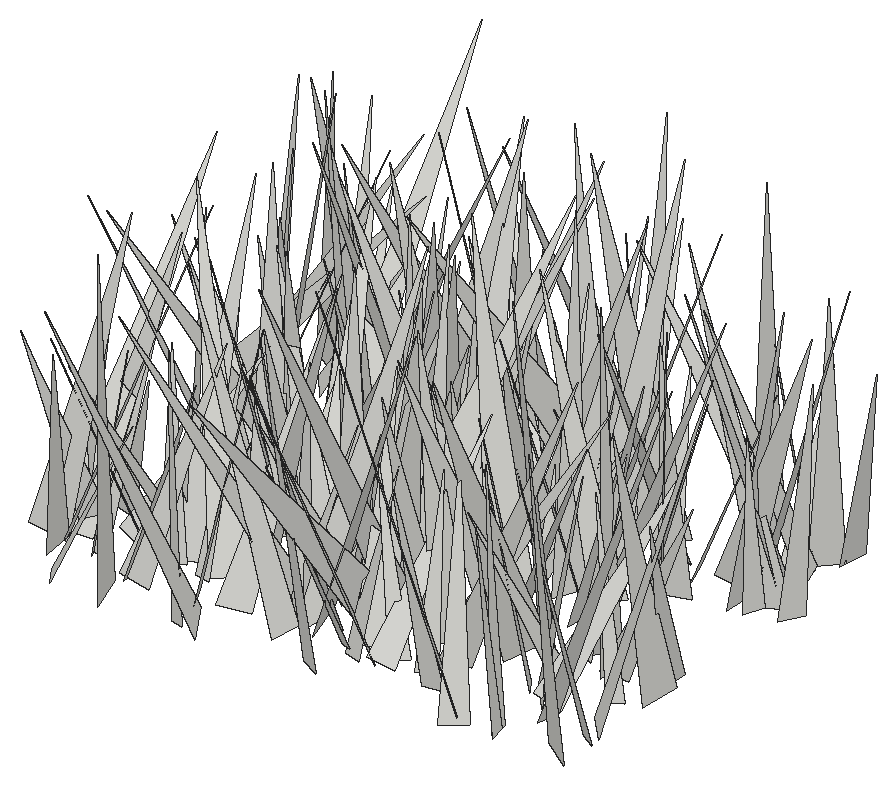
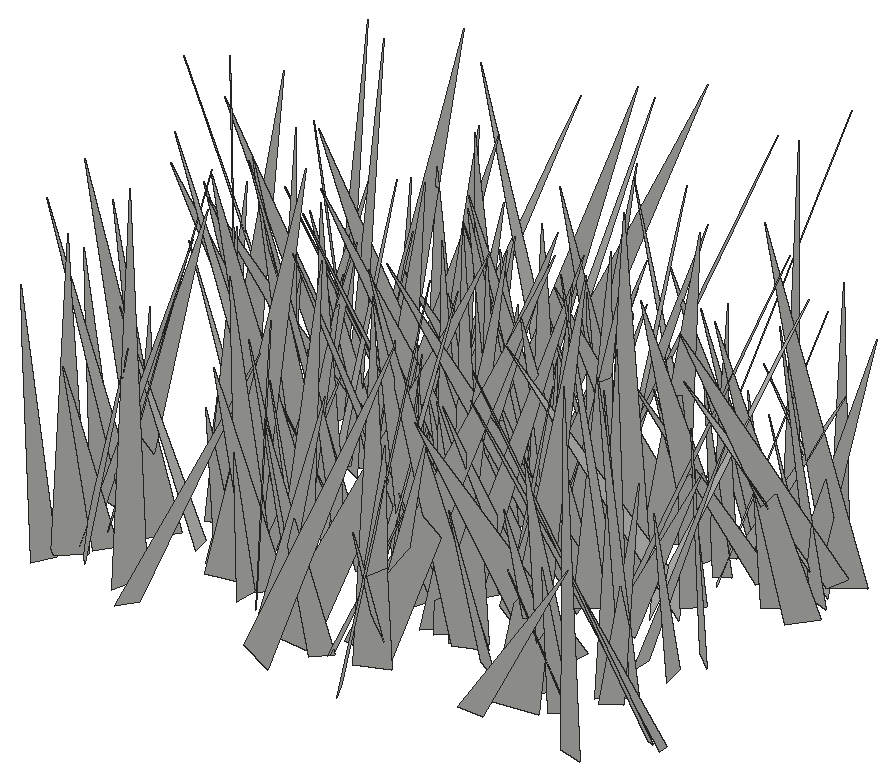
# SketchUp Ruby script. Lengths in inches.
U = 1.inch
M = Sketchup.active_model
def pt(a) = Geom::Point3d.new(a.map { |v| v * U })
def face(e, loops, mat)
  f = e.add_face(loops[0].map { |a| pt(a) })
  loops[1..].each { |l| e.add_face(l.map { |a| pt(a) }).erase! }
  f.material = f.back_material = mat if mat
  f
end
# faces: each face lists its corners as indices into pts; further lists are holes
def faces(e, pts, list, mat = nil) = list.each { |f| face(e, (f[0].is_a?(Array) ? f : [f]).map { |l| l.map { |i| pts[i] } }, mat) }
# xy, xz, yz: faces in a plane at the given z, y or x. An outline is a flat list of corners, or four numbers for a rectangle; further outlines are holes
def ring(l) = l.size == 4 ? [[l[0], l[1]], [l[2], l[1]], [l[2], l[3]], [l[0], l[3]]] : l.each_slice(2).to_a
def flat(e, list, mat, &to3) = list.each { |f| face(e, (f[0].is_a?(Array) ? f : [f]).map { |l| ring(l).map { |u, v| to3.(u, v) } }, mat) }
def xy(e, z, list, mat = nil) = flat(e, list, mat) { |x, y| [x, y, z] }
def xz(e, y, list, mat = nil) = flat(e, list, mat) { |x, z| [x, y, z] }
def yz(e, x, list, mat = nil) = flat(e, list, mat) { |y, z| [x, y, z] }
def lines(e, pts, list) = list.each { |a, b| e.add_line(pt(pts[a]), pt(pts[b])) }
# prism: a flat outline (further loops are holes) pulled along v
def prism(e, loops, v, mat = nil)
  f = face(e, loops, mat); d = Geom::Vector3d.new(v.map { |x| x * U })
  f.pushpull(f.normal.samedirection?(d) ? d.length : -d.length)
end
def box(e, o, s, mat = nil) = prism(e, [[o, [o[0] + s[0], o[1], o[2]], [o[0] + s[0], o[1] + s[1], o[2]], [o[0], o[1] + s[1], o[2]]]], [0, 0, s[2]], mat)
def at(x, y, z, deg = 0) = Geom::Transformation.translation(pt([x, y, z])) * Geom::Transformation.rotation(ORIGIN, Z_AXIS, deg.degrees)
def axes(o, x, y, z) = Geom::Transformation.new([*x, 0, *y, 0, *z, 0, *pt(o).to_a, 1])
def part(name) = M.definitions.add(name)
# library, detail: a bought-in or finely detailed component or shape, given as its bounding box
def library(name, o, s) = part(name).tap { |d| box(d.entities, o, s) }
def detail(e, o, s) = box(e.add_group.entities, o, s)
def put(e, d, t, mat = nil) = e.add_instance(d, t).tap { |i| i.material = mat if mat }
def group(e, t, mat = nil) = e.add_group.tap { |g| g.transformation = t; g.material = mat if mat }.entities
root = M.entities
c1 = part("fur_instance\#9")
p = [[0.8125,0,1.79],[0.67,-0.02,1.48],[0,-0.11,0],[0,0.11,0]]
faces(c1.entities,p,[[0,1,2,3]])
put(root,c1,axes([534.78,5.64,-21.86],[-6.5639,-4.29471,0.69968],[-4.06333,6.50273,1.7952],[1.55674,-1.13527,7.63588]))
put(root,c1,axes([530.92,5.27,-21.86],[6.72646,1.81373,2.96578],[2.30607,-7.16166,-0.85049],[-2.60144,-1.65881,6.91459]))
put(root,c1,axes([540.06,9.92,-21.86],[5.96387,-5.74764,0.45925],[-4.68382,-5.21453,-4.43673],[-3.36276,-2.93042,6.99418]))
put(root,c1,axes([540.83,7.86,-21.86],[-4.50054,-5.78959,0.45114],[-5.68851,4.51005,1.13049],[1.1678,-0.3432,7.24542]))
put(root,c1,axes([550.6875,6.2,-21.86],[-3.10043,-5.65859,2.0595],[-5.81568,3.41455,0.62657],[1.56175,1.48157,6.42182]))
put(root,c1,axes([527.36,6.95,-21.86],[5.21183,-0.69159,1.00189],[-0.40075,-5.13378,-1.45906],[-1.14955,-1.3458,5.051]))
put(root,c1,axes([528.53,5.1,-21.86],[3.11612,2.14822,0.04863],[2.13222,-3.08072,-0.53874],[0.26618,-0.47091,3.74631]))
put(root,c1,axes([539.89,5.63,-21.86],[-3.61019,-4.99925,2.09321],[-5.40705,3.49453,-0.97958],[0.37125,2.28107,6.08822]))
put(root,c1,axes([536.85,9.12,-21.86],[-6.99156,-3.62516,0.34789],[-3.32905,6.6672,2.57109],[1.47657,-2.13338,7.444]))
put(root,c1,axes([548.125,6.03,-21.86],[-3.70453,-1.18645,1.17686],[-1.32576,3.8289,-0.31316],[1.01735,0.66938,3.87726]))
put(root,c1,axes([546.48,5.59,-21.86],[-3.13208,3.88614,1.48189],[4.03166,3.29255,-0.11327],[1.02167,-1.07935,4.98991]))
put(root,c1,axes([534.21,5.15,-21.86],[2.11114,4.26728,1.69749],[4.08085,-2.60007,1.46097],[-2.10662,-0.76029,4.53125]))
put(root,c1,axes([544.27,7.17,-21.86],[0.17037,-4.40384,1.04145],[-4.5148,-0.2364,-0.26107],[-0.30825,1.02847,4.3994]))
put(root,c1,axes([545.93,6.41,-21.86],[-6.31099,-5.2237,1.0112],[-5.28027,5.95593,-2.18722],[-0.65451,2.31907,7.89505]))
put(root,c1,axes([533.68,6.97,-21.86],[5.91305,2.63208,1.30513],[2.84881,-5.85376,-1.10147],[-0.71801,-1.54954,6.37799]))
put(root,c1,axes([547.97,6.27,-21.86],[-4.75488,-0.89522,1.48594],[-1.16705,4.85843,-0.80746],[1.28353,1.10117,4.77057]))
put(root,c1,axes([539.92,7.66,-21.86],[-2.11494,-3.26023,0.3236],[-3.25153,2.04149,-0.68318],[-0.40176,0.64034,3.82562]))
put(root,c1,axes([530.75,6.95,-21.86],[4.6292,0.17151,0.50537],[0.17521,-4.6565,-0.02456],[-0.5041,-0.0434,4.63231]))
put(root,c1,axes([531.11,6.63,-21.86],[-0.2633,5.21725,2.01289],[5.21535,0.95622,-1.79623],[2.01778,-1.79073,4.90536]))
put(root,c1,axes([527.55,8.98,-21.86],[3.42862,-3.42654,1.21049],[-3.04602,-3.61734,-1.61199],[-1.98197,-0.36822,4.57144]))
put(root,c1,axes([550.95,7.64,-21.86],[-3.27995,-3.84872,1.10692],[-4.00472,3.15616,-0.89264],[0.01123,1.42196,4.97734]))
put(root,c1,axes([538.19,8.56,-21.86],[7.97506,1.59703,0.67128],[1.71117,-7.75527,-1.87893],[-0.27022,-1.97686,7.91339]))
put(root,c1,axes([537.64,7.04,-21.86],[-7.05219,-0.0174,0.36445],[-0.04272,7.04446,-0.49029],[0.36236,0.49184,7.03515]))
put(root,c1,axes([530.27,10.26,-21.86],[-4.13321,-3.41194,0.20507],[-3.07913,3.85633,2.10107],[1.48403,-1.5014,4.93054]))
put(root,c1,axes([540.35,10.58,-21.86],[0.33917,-8.30019,0.61155],[-8.21231,-0.43312,-1.32383],[-1.35096,0.54903,8.20095]))
put(root,c1,axes([530.93,7.98,-21.86],[-3.23089,-3.2407,0.20186],[-3.09319,2.98531,-1.58167],[-0.98745,1.25194,4.29408]))
put(root,c1,axes([526.48,7.53,-21.86],[1.86303,-6.4471,2.90273],[-6.99316,-1.23765,1.73947],[1.04242,3.21946,6.48153]))
put(root,c1,axes([538.75,8.64,-21.86],[-2.94659,-4.28728,0.79485],[-4.35538,2.84813,-0.78348],[-0.2081,1.09651,5.14289]))
put(root,c1,axes([545.16,11.39,-21.86],[6.488,-4.94571,0.82766],[-4.48999,-6.33233,-2.64212],[-2.23271,-1.63731,7.71838]))
put(root,c1,axes([542.06,8.05,-21.86],[-1.79664,3.17113,0.9039],[3.29721,1.71578,0.53432],[-0.03822,-1.04932,3.60534]))
put(root,c1,axes([528.65,7.34,-21.86],[2.93854,2.24557,1.05284],[2.03507,-3.11619,0.96641],[-1.41759,0.18132,3.56983]))
put(root,c1,axes([547.59,9.15,-21.86],[4.29125,3.34973,1.68987],[3.74545,-3.97458,-1.63261],[-0.21889,-2.33948,5.19327]))
put(root,c1,axes([538.01,8.5,-21.86],[-4.77809,0.40303,0.49366],[0.4272,4.79644,0.21897],[0.47289,-0.2608,4.79006]))
put(root,c1,axes([537.06,8.1,-21.86],[2.48119,3.58815,0.88423],[3.68479,-2.32113,-0.92071],[0.2811,-1.24521,4.2642]))
put(root,c1,axes([543.37,7.96,-21.86],[-2.54986,2.80817,1.27437],[2.87177,2.76487,-0.34653],[1.12374,-0.69377,3.77724]))
put(root,c1,axes([538.08,10.45,-21.86],[2.95419,-3.46444,1.08183],[-2.95275,-3.10527,-1.88109],[-2.11044,-0.50488,4.14621]))
put(root,c1,axes([531.36,8.52,-21.86],[1.67153,-3.68103,1.97281],[-4.08391,-1.88531,-0.05752],[-0.87388,1.76964,4.04237]))
put(root,c1,axes([528.93,7.34,-21.86],[1.45638,3.8911,0.37542],[3.87774,-1.48869,0.38679],[-0.49475,-0.21394,4.13668]))
put(root,c1,axes([546.92,10.95,-21.86],[-4.05266,-1.43323,0.72397],[-1.06557,3.87082,1.69814],[1.20119,-1.40176,3.94899]))
put(root,c1,axes([546.9,9.44,-21.86],[-3.48684,-2.54111,1.02639],[-2.66037,3.53733,-0.28017],[0.65812,0.83597,4.30544]))
put(root,c1,axes([526.6,9.09,-21.86],[2.41252,4.65389,1.89869],[5.02303,-2.30836,-0.72433],[-0.1815,-2.02404,5.19175]))
put(root,c1,axes([530.49,9.68,-21.86],[0.50859,-3.54434,0.97529],[-3.61365,-0.30136,0.78924],[0.67458,1.05784,3.49258]))
put(root,c1,axes([540.58,8.12,-21.86],[-2.22109,4.73282,1.14399],[4.81333,2.32397,-0.26934],[0.73496,-0.91711,5.22114]))
put(root,c1,axes([542.74,10.16,-21.86],[3.54462,-5.56954,2.15269],[-5.7416,-3.86654,-0.54956],[-1.63946,1.49942,6.57891]))
put(root,c1,axes([527.76,10.34,-21.86],[0.50493,-3.90237,0.56248],[-3.75126,-0.30094,1.27958],[1.21364,0.69337,3.72104]))
put(root,c1,axes([541.68,7.43,-21.86],[-1.38897,4.86037,0.26759],[4.61521,1.40338,-1.53442],[1.54748,0.17706,4.81643]))
put(root,c1,axes([534.17,9.83,-21.86],[6.74375,-1.56753,0.95704],[-1.61805,-6.79399,0.27364],[-0.86892,0.48558,6.91813]))
put(root,c1,axes([532.88,8.29,-21.86],[1.32341,3.79294,0.4756],[3.74321,-1.38791,0.65276],[-0.77522,-0.22654,3.9638]))
put(root,c1,axes([534.07,11.92,-21.86],[-4.79038,-5.44103,1.36632],[-5.2062,4.98101,1.5825],[2.08977,-0.06337,7.07448]))
put(root,c1,axes([543.89,8.81,-21.86],[6.12264,-2.56902,1.18593],[-2.80714,-5.86992,1.77677],[-0.35534,2.10644,6.39763]))
put(root,c1,axes([543.74,12.12,-21.86],[4.33462,-5.23656,1.50263],[-4.77333,-4.57611,-2.17783],[-2.62578,-0.3257,6.43953]))
put(root,c1,axes([548.82,8.06,-21.86],[6.71372,1.26121,1.18447],[0.98901,-6.69183,1.51954],[-1.41968,1.3025,6.66001]))
put(root,c1,axes([540.61,7.15,-21.86],[3.46655,5.88623,0.70358],[5.62008,-3.5225,1.77941],[-1.8861,0.32244,6.59533]))
put(root,c1,axes([536.04,9.95,-21.86],[0.99186,4.25892,2.03749],[4.71935,-0.95274,-0.30591],[-0.13232,-2.05608,4.36218]))
put(root,c1,axes([533.63,9.02,-21.86],[-4.74257,5.72398,1.5327],[5.90767,4.72004,0.65254],[0.46105,-1.60076,7.40474]))
put(root,c1,axes([550.99,11.6875,-21.86],[5.89812,-2.41371,1.85981],[-1.99813,-6.12286,-1.60962],[-2.30052,-0.87028,6.16628]))
put(root,c1,axes([550.64,8.54,-21.86],[5.3088,5.05785,1.00754],[5.10033,-5.36326,0.04959],[-0.76398,-0.65873,7.33231]))
put(root,c1,axes([535.15,7.22,-21.86],[-4.70627,4.28235,1.06672],[3.70191,4.67966,-2.45399],[2.40255,1.178,5.87073]))
put(root,c1,axes([540.34,11.71,-21.86],[-4.48343,0.78051,2.64752],[1.64873,4.80743,1.37477],[2.21365,-1.99978,4.33824]))
put(root,c1,axes([545.76,11.88,-21.86],[-3.953,-6.85404,2.35159],[-6.87911,4.39144,1.23577],[2.27722,1.36799,7.81517]))
put(root,c1,axes([529.01,9.04,-21.86],[0.32449,4.79651,0.65441],[4.29347,0.01783,-2.25961],[2.23626,-0.73022,4.24334]))
put(root,c1,axes([548.07,8.9375,-21.86],[-0.77489,5.32124,0.74593],[4.8544,1.01638,-2.20776],[2.30365,-0.35187,4.90325]))
put(root,c1,axes([529.91,12.04,-21.86],[2.72527,-3.47225,0.02549],[-3.46346,-2.7159,0.33551],[0.24824,0.22715,4.40125]))
put(root,c1,axes([536.96,11.52,-21.86],[3.71508,-1.29272,0.27873],[-1.28155,-3.72443,-0.19222],[-0.32626,-0.0905,3.92887]))
put(root,c1,axes([526.21,10.46,-21.86],[3.16186,-4.77933,2.12939],[-5.21892,-2.70344,1.68164],[0.37303,2.68757,5.47827]))
put(root,c1,axes([527.26,7.59,-21.86],[5.40862,3.75774,0.29196],[3.28966,-4.95573,2.84217],[-1.83956,2.18614,5.94103]))
put(root,c1,axes([550.65,12.85,-21.86],[4.29129,-1.7599,0.57931],[-1.53313,-4.1935,-1.38278],[-1.04037,-1.07949,4.42723]))
put(root,c1,axes([550,10.38,-21.86],[-0.43735,3.78387,0.74816],[3.7266,0.2203,1.06426],[-0.99494,-0.83814,3.65736]))
put(root,c1,axes([538.03,12.92,-21.86],[2.29516,-7.21123,1.1617],[-7.23425,-2.07612,1.40519],[1.00849,1.5189,7.43607]))
put(root,c1,axes([531.05,13.0625,-21.86],[-5.75391,-4.14909,0.07824],[-4.14913,5.75437,0.02082],[0.07564,0.02888,7.0938]))
put(root,c1,axes([548.73,11.93,-21.86],[2.75762,-4.13306,0.47465],[-3.98702,-2.46295,1.71739],[1.18791,1.32801,4.66232]))
put(root,c1,axes([531.58,8.9375,-21.86],[-5.90287,3.96424,1.22936],[3.5461,5.92766,-2.08769],[2.15678,1.10365,6.7971]))
put(root,c1,axes([542.28,11.16,-21.86],[4.10846,4.74791,0.21399],[4.46685,-3.7608,-2.31765],[1.62348,-1.66782,5.83529]))
put(root,c1,axes([543.86,12.18,-21.86],[5.27208,0.02621,0.0042],[0.02652,-5.23568,-0.61848],[-0.0011,-0.61849,5.23574]))
put(root,c1,axes([527.07,8.03,-21.86],[-5.0261,5.87636,0.71878],[5.2638,4.86732,-2.98524],[2.70938,1.44485,7.13314]))
put(root,c1,axes([533.44,13.21,-21.86],[2.7716,-4.32676,0.73791],[-4.29866,-2.85215,-0.57784],[-0.88707,0.30254,5.10575]))
put(root,c1,axes([536.59,12.125,-21.86],[-1.98157,5.41612,3.08152],[6.10168,2.34277,-0.19399],[1.26474,-2.81671,5.76397]))
put(root,c1,axes([536.55,10.88,-21.86],[0.16131,6.95669,2.04491],[7.08472,0.28432,-1.5261],[1.54396,-2.03146,6.78915]))
put(root,c1,axes([538.43,11.3,-21.86],[-1.99924,6.11191,2.2816],[6.3463,2.375,-0.80119],[1.51181,-1.88733,6.38047]))
put(root,c1,axes([532.84,12.125,-21.86],[5.17413,-4.7343,3.23528],[-5.24163,-5.67192,0.08293],[-2.32507,2.25121,7.01272]))
put(root,c1,axes([535.25,12.21,-21.86],[-4.86777,3.35697,1.6535],[3.6105,4.92638,0.62739],[0.98366,-1.46972,5.8797]))
put(root,c1,axes([530.53,16.49,-21.86],[-6.95908,-3.88864,0.42907],[-3.38575,6.42493,3.31533],[1.96017,-2.70799,7.24975]))
put(root,c1,axes([548.41,12.17,-21.86],[-6.67663,-0.80436,2.4344],[-1.05353,7.05179,-0.55944],[2.33738,0.88086,6.7016]))
put(root,c1,axes([549.54,13.53,-21.86],[6.08028,3.66314,2.96745],[4.34842,-6.22849,-1.22118],[-1.82087,-2.64225,6.99265]))
put(root,c1,axes([532.6875,14.28,-21.86],[4.51111,-4.76568,1.07484],[-4.75985,-4.61702,-0.49408],[-1.1004,0.43419,6.54353]))
put(root,c1,axes([546.88,12.46,-21.86],[2.00613,4.44684,1.43472],[4.67253,-1.91449,-0.59961],[-0.01581,-1.5549,4.84142]))
put(root,c1,axes([535.28,13.72,-21.86],[3.93197,-0.07434,1.3447],[0.21137,-4.06439,-0.84276],[-1.33006,-0.86567,3.84131]))
put(root,c1,axes([543.21,13.45,-21.86],[-2.98198,-2.20876,0.85448],[-2.34628,2.94214,-0.58291],[0.32208,0.98295,3.66484]))
put(root,c1,axes([545.26,14.48,-21.86],[6.29896,-1.22347,0.37639],[-1.1888,-6.29213,-0.55798],[-0.47466,-0.47719,6.39237]))
put(root,c1,axes([539.03,12.3,-21.86],[-6.72767,0.28008,1.7782],[-0.11729,6.79671,-1.51427],[1.7963,1.49276,6.56102]))
put(root,c1,axes([535.36,12.83,-21.86],[3.71678,-0.58843,1.31141],[-0.99782,-3.67326,1.17982],[-1.0346,1.42876,3.57333]))
put(root,c1,axes([543.28,16.53,-21.86],[-4.09949,-5.26965,1.04192],[-4.89422,4.20438,2.00758],[2.21389,-0.46331,6.36747]))
put(root,c1,axes([540.02,12.07,-21.86],[-6.09704,1.94582,1.05535],[1.61207,6.02238,-1.79053],[1.51697,1.42075,6.14444]))
put(root,c1,axes([539.18,14.87,-21.86],[-3.57828,-1.18752,0.86435],[-1.11493,3.67791,0.43741],[0.95617,-0.15551,3.74473]))
put(root,c1,axes([542.14,14.3125,-21.86],[-5.03128,5.10175,2.45438],[5.52933,5.13327,0.66454],[1.21582,-2.23324,7.13442]))
put(root,c1,axes([547.07,12.45,-21.86],[6.92746,0.46404,1.30725],[0.06508,-6.75935,2.05449],[-1.38564,2.00246,6.63205]))
put(root,c1,axes([534.96,12.59,-21.86],[-3.90742,5.66938,0.63215],[5.60395,3.95813,-0.85923],[1.06639,-0.02677,6.83166]))
put(root,c1,axes([538.68,16.57,-21.86],[1.6071,-3.85332,0.26864],[-3.82652,-1.62792,-0.45895],[-0.52725,0.06941,4.14972]))
put(root,c1,axes([538.12,12.82,-21.86],[0.28527,8.21503,1.11931],[7.94931,0.04717,-2.37217],[2.35543,-1.15413,7.87026]))
put(root,c1,axes([538.6,16.52,-21.86],[1.94153,-7.03493,2.68991],[-6.84514,-2.80689,-2.40016],[-3.14163,1.7682,6.89195]))
put(root,c1,axes([527.22,14.83,-21.86],[2.79154,3.79561,1.789],[3.98615,-3.06992,0.29332],[-1.31064,-1.25251,4.70248]))
put(root,c1,axes([530.77,15.09,-21.86],[-2.74524,3.88345,0.46197],[3.73915,2.44095,1.70042],[-1.14601,-1.33847,4.4414]))
put(root,c1,axes([541.78,15.02,-21.86],[1.87721,3.55983,2.07479],[3.45548,-2.60202,1.33802],[-2.2443,-1.02868,3.79553]))
put(root,c1,axes([547.1,15.27,-21.86],[4.65489,2.00226,0.76997],[2.06003,-4.68544,-0.26978],[-0.59848,-0.55448,5.06006]))
put(root,c1,axes([530.43,12.11,-21.86],[6.17595,4.1917,0.11311],[3.92557,-5.85042,2.46738],[-1.47413,1.98185,7.04448]))
put(root,c1,axes([537.7,15.79,-21.86],[-2.59622,-3.87524,1.56211],[-4.17566,2.47102,-0.8099],[0.14666,1.75346,4.59368]))
put(root,c1,axes([528.72,16.52,-21.86],[-4.93591,-0.64757,0.62999],[-0.58328,4.95621,0.52453],[0.68994,-0.44273,4.95049]))
put(root,c1,axes([534.81,14.99,-21.86],[4.39475,-2.24157,1.41228],[-2.61052,-4.13054,1.56743],[-0.4521,2.06082,4.67778]))
put(root,c1,axes([538.23,16.8125,-21.86],[2.32734,-2.83374,0.7234],[-2.82694,-2.41664,-0.37171],[-0.74954,0.31569,3.64807]))
put(root,c1,axes([545.21,16.04,-21.86],[1.40362,-5.52471,3.15038],[-5.88186,-2.35471,-1.50878],[-2.41887,2.51999,5.49692]))
put(root,c1,axes([534.74,16.63,-21.86],[-2.18314,-4.32344,1.23175],[-4.48368,1.99494,-0.94459],[-0.32548,1.51774,4.75036]))
put(root,c1,axes([543.76,15.58,-21.86],[-6.82221,1.72842,2.33339],[1.55801,7.20655,-0.7829],[2.45045,0.23004,6.99407]))
put(root,c1,axes([542.18,16.08,-21.86],[2.36408,2.77163,0.06713],[2.67068,-2.25294,-1.03299],[0.74428,-0.71945,3.49339]))
put(root,c1,axes([535.73,18.27,-21.86],[-2.92587,-7.18113,1.16279],[-7.26033,2.80394,-0.95233],[-0.45638,1.43204,7.69561]))
put(root,c1,axes([536.11,14.49,-21.86],[-6.55777,-1.69063,0.96933],[-1.94723,5.82112,-3.02077],[0.07829,3.17151,6.06115]))
put(root,c1,axes([535.39,18.82,-21.86],[6.03142,-3.81553,0.06105],[-3.78285,-5.99326,-0.84318],[-0.50203,-0.68018,7.08699]))
put(root,c1,axes([533.87,15.81,-21.86],[3.01287,6.59159,3.14785],[6.68601,-3.85992,1.68335],[-2.94198,-2.02171,7.04931]))
put(root,c1,axes([533.34,13.74,-21.86],[8.13391,1.72844,0.70897],[1.41113,-7.75982,2.72846],[-1.22428,2.53935,7.85515]))
put(root,c1,axes([537.02,14.96,-21.86],[4.52009,6.67395,0.30614],[6.59904,-4.40227,-1.46264],[1.04307,-1.07006,7.92676]))
put(root,c1,axes([534.51,19.1,-21.86],[1.32188,-7.44707,0.58602],[-7.30684,-1.16527,1.67389],[1.55318,0.85612,7.37593]))
put(root,c1,axes([528.08,18.98,-21.86],[5.72206,-2.67718,0.30846],[-2.55509,-5.6197,-1.37653],[-0.85672,-1.12072,6.16558]))
put(root,c1,axes([546.83,17.78,-21.86],[1.69924,-5.28596,1.58911],[-5.50046,-1.7602,0.02657],[-0.46001,1.5213,5.5523]))
put(root,c1,axes([527.34,16.39,-21.86],[-3.53887,0.08812,1.47041],[-0.2173,3.75324,-0.74791],[1.45693,0.77383,3.46005]))
put(root,c1,axes([542.99,18.49,-21.86],[-1.08369,-5.40972,1.03151],[-5.49173,1.14023,0.21038],[0.41232,0.96864,5.51318]))
put(root,c1,axes([529.18,16.97,-21.86],[6.97385,3.06548,2.09729],[3.25235,-7.19468,-0.2986],[-1.79388,-1.12684,7.61201]))
put(root,c1,axes([544.15,18.56,-21.86],[-3.71284,-0.24914,0.82183],[0.046,3.58403,1.29433],[0.85753,-1.27095,3.48884]))
put(root,c1,axes([529.4,16.54,-21.86],[3.68214,4.39884,2.0354],[4.4735,-4.06815,0.69917],[-1.86561,-1.07294,5.69378]))
put(root,c1,axes([535.99,18.84,-21.86],[-6.33507,2.2676,3.27677],[3.13305,6.63723,1.4641],[2.46237,-2.61105,6.56746]))
put(root,c1,axes([544.94,20.31,-21.86],[-1.67702,-6.45132,0.05531],[-6.32349,1.655,1.30744],[1.27907,-0.27646,6.53625]))
put(root,c1,axes([535.02,18.27,-21.86],[2.13927,-3.81253,0.27989],[-3.71667,-1.99926,1.17453],[0.89447,0.81104,4.21098]))
put(root,c1,axes([538.91,19.21,-21.86],[2.00782,-4.43373,0.05819],[-4.43409,-2.00742,0.0429],[0.01508,0.0707,4.86698]))
put(root,c1,axes([540.54,17.53,-21.86],[4.58596,6.39713,1.96066],[6.63658,-4.04695,-2.31874],[0.85046,-2.91504,7.52182]))
put(root,c1,axes([536.1875,16.11,-21.86],[-3.10832,3.75001,0.92239],[3.63037,3.24121,-0.94342],[1.31674,-0.08395,4.77852]))
put(root,c1,axes([533.9,16.125,-21.86],[4.95008,1.27612,1.12304],[0.89586,-4.89693,1.61571],[-1.4447,1.33589,4.84988]))
put(root,c1,axes([543.12,17.74,-21.86],[7.89024,2.57718,0.73013],[2.64489,-7.85516,-0.85554],[-0.42369,-1.04189,8.25626]))
put(root,c1,axes([537.72,17.0625,-21.86],[1.56469,4.5597,1.40699],[4.65343,-1.78584,0.61247],[-1.05645,-1.11294,4.78163]))
put(root,c1,axes([542.04,16.61,-21.86],[0.07202,5.27236,0.64208],[5.29211,-0.12578,0.43929],[-0.45123,-0.63374,5.25452]))
put(root,c1,axes([549.67,18.71,-21.86],[3.35457,-1.66316,1.27005],[-1.64462,-3.57909,-0.343],[-1.29397,0.23728,3.72849]))
put(root,c1,axes([538.78,17.1,-21.86],[-4.01234,0.85775,1.7856],[0.34464,4.27421,-1.27879],[1.95072,1.00913,3.89863]))
put(root,c1,axes([549.88,20.28,-21.86],[-5.81163,-3.8947,1.27527],[-3.71182,5.94036,1.22659],[1.73708,-0.33677,6.88761]))
put(root,c1,axes([527.82,19.35,-21.86],[3.23004,-2.47849,1.2151],[-2.38486,-3.44753,-0.69249],[-1.3899,0.15559,4.01205]))
put(root,c1,axes([536.91,21.85,-21.86],[1.87232,-8.06563,0.81969],[-7.60481,-2.03883,-2.69107],[-2.80947,0.14362,7.83059]))
put(root,c1,axes([547.92,19.78,-21.86],[2.64878,-6.42579,1.07864],[-6.29914,-2.22772,2.19734],[1.66585,1.79353,6.59382]))
put(root,c1,axes([538.09,19.18,-21.86],[4.40996,1.53054,2.75088],[1.88618,-5.07543,-0.19988],[-2.52036,-1.1203,4.66373]))
put(root,c1,axes([543.88,17.19,-21.86],[6.54564,-3.57049,3.76512],[-4.66006,-6.71077,1.73761],[-2.28219,3.46223,7.25083]))
put(root,c1,axes([548.91,18.78,-21.86],[6.13024,0.22864,1.74835],[0.20896,-6.37456,0.10097],[-1.75081,0.03976,6.13367]))
put(root,c1,axes([528.22,17.81,-21.86],[2.58836,6.22661,1.98748],[6.38761,-2.86286,0.6503],[-1.38536,-1.56644,6.71174]))
put(root,c1,axes([539.53,22.99,-21.86],[4.76692,-6.38187,0.99404],[-5.33821,-4.5884,-3.85875],[-3.63592,-1.6304,6.96863]))
put(root,c1,axes([551.07,19.1,-21.86],[4.44334,-1.86269,1.64457],[-2.02269,-4.66849,0.17731],[-1.44323,0.80817,4.81471]))
put(root,c1,axes([538.89,19.32,-21.86],[-5.72763,-4.55632,1.57593],[-4.80185,5.61014,-1.23206],[0.43111,1.95337,7.21442]))
put(root,c1,axes([550.16,19.3,-21.86],[-0.65544,-6.57541,2.82853],[-6.91722,-0.14862,-1.94837],[-1.84083,2.89967,6.31422]))
put(root,c1,axes([536.3,18.17,-21.86],[3.571,6.90444,0.98118],[6.89309,-3.32732,-1.67343],[1.05801,-1.62595,7.59098]))
put(root,c1,axes([546.39,19.48,-21.86],[4.46845,1.48023,0.19389],[1.49287,-4.43008,-0.58427],[0.00126,-0.6156,4.67084]))
put(root,c1,axes([530.3,21.6875,-21.86],[1.76512,-7.95634,1.31885],[-8.03843,-1.84494,-0.37166],[-0.65291,1.20466,8.14131]))
put(root,c1,axes([544.05,20.77,-21.86],[2.92408,-7.38877,2.72238],[-7.56214,-3.44459,-1.22649],[-2.19528,2.02396,7.85111]))
put(root,c1,axes([537.52,17.57,-21.86],[5.43527,-3.00495,4.38513],[-4.48513,-5.95873,1.47596],[-2.85354,3.64214,6.0327]))
put(root,c1,axes([534.27,19.28,-21.86],[0.54119,7.40359,2.44886],[7.61955,0.0202,-1.74498],[1.65906,-2.50787,7.21533]))
put(root,c1,axes([549.71,21.8,-21.86],[-5.8236,-1.97497,1.08531],[-1.72724,5.8434,1.36532],[1.44743,-0.9731,5.99589]))
put(root,c1,axes([542.29,19.3,-21.86],[-7.50799,1.69583,1.59774],[1.55933,7.66276,-0.80567],[1.73121,0.45255,7.65484]))
put(root,c1,axes([524.33,20.73,-21.86],[4.7067,5.43888,0.18038],[4.50837,-3.76361,-4.15655],[3.04771,-2.83211,5.87006]))
put(root,c1,axes([545.14,19.62,-21.86],[-2.61192,2.51011,0.78878],[2.46687,2.72278,-0.49597],[0.91509,-0.17543,3.58843]))
put(root,c1,axes([540.54,20.83,-21.86],[3.90059,1.73334,0.99556],[1.91928,-3.85762,-0.80331],[-0.55855,-1.15086,4.19211]))
put(root,c1,axes([548.92,19.97,-21.86],[6.30339,2.19635,1.13005],[2.22882,-6.39265,-0.00763],[-1.06457,-0.37914,6.67507]))
put(root,c1,axes([537.39,20.37,-21.86],[-4.286,2.05614,0.85108],[2.13965,4.31523,0.34994],[0.6115,-0.68765,4.74078]))
put(root,c1,axes([524.98,20.66,-21.86],[5.32286,5.30667,0.20638],[4.93366,-4.8331,-2.97258],[1.96528,-2.23975,6.90343]))
put(root,c1,axes([530.56,19.54,-21.86],[-1.52341,4.48001,0.30788],[4.47725,1.54034,-0.26007],[0.34571,-0.20714,4.72479]))
put(root,c1,axes([537.86,22.74,-21.86],[-3.34335,-1.51871,0.13226],[-1.40215,3.18862,1.16988],[0.59829,-1.01398,3.48078]))
put(root,c1,axes([541.77,19.76,-21.86],[1.82838,5.64567,1.15342],[5.69001,-1.95997,0.57384],[-0.90985,-0.91206,5.90655]))
put(root,c1,axes([536.13,22.57,-21.86],[1.85268,-6.56464,1.39244],[-6.70428,-1.74747,0.68181],[0.2934,1.52239,6.78691]))
put(root,c1,axes([542.36,21.36,-21.86],[-4.40906,-3.22075,2.19411],[-3.50304,4.72714,-0.10035],[1.70765,1.38134,5.45921]))
put(root,c1,axes([530.1,19.59,-21.86],[-5.38629,2.97439,0.98855],[2.72826,5.41671,-1.43257],[1.54299,0.80541,5.98388]))
put(root,c1,axes([527.4,21.79,-21.86],[3.3764,2.66955,0.1135],[2.47122,-3.05035,-1.76859],[1.01611,-1.452,3.92412]))
put(root,c1,axes([528.875,20.97,-21.86],[-1.83169,3.1238,0.57494],[3.14275,1.87858,-0.19441],[0.4602,-0.39568,3.61599]))
put(root,c1,axes([532.76,20.17,-21.86],[1.48106,4.37962,0.44895],[4.22706,-1.54701,1.14671],[-1.23071,-0.04293,4.4788]))
put(root,c1,axes([549.625,22.91,-21.86],[-3.8078,3.44308,3.43375],[4.19662,4.52997,0.11149],[2.45637,-2.40193,5.13242]))
put(root,c1,axes([526.61,23.1875,-21.86],[-2.31612,-6.1908,2.36322],[-6.27799,2.85121,1.3163],[2.12077,1.67923,6.47748]))
put(root,c1,axes([535.98,24.6,-21.86],[-6.24986,-4.52728,1.84324],[-4.17742,6.50052,1.80193],[2.5383,-0.44892,7.504]))
put(root,c1,axes([542.4375,20.55,-21.86],[-3.17134,4.85922,0.78552],[4.77597,3.26378,-0.90795],[1.19131,-0.14895,5.73106]))
put(root,c1,axes([537.66,20.76,-21.86],[-3.60755,4.52257,0.00535],[4.517,3.60276,0.29145],[-0.22451,-0.18592,5.77782]))
put(root,c1,axes([542.83,20.79,-21.86],[-7.20595,2.28011,2.02761],[1.9171,7.42879,-1.54068],[2.37378,0.922,7.39939]))
put(root,c1,axes([530.9,18.14,-21.86],[-6.04626,5.73242,0.3376],[5.11125,5.59588,-3.47751],[2.61721,2.31459,7.57131]))
put(root,c1,axes([548.93,21.77,-21.86],[-2.21972,3.26489,1.22418],[3.2229,2.47495,-0.75684],[1.3308,-0.54808,3.87477]))
put(root,c1,axes([546.69,23.18,-21.86],[7.21029,-1.27081,2.71678],[-1.16788,-7.70491,-0.50453],[-2.76259,-0.05954,7.30402]))
put(root,c1,axes([549.29,22.56,-21.86],[2.56501,3.25674,2.5986],[3.3721,-3.41499,0.95138],[-2.44704,-1.29222,4.03491]))
put(root,c1,axes([550.11,23.77,-21.86],[4.83385,-1.43847,0.54232],[-1.36908,-4.84202,-0.64023],[-0.69925,-0.46374,5.00254]))
put(root,c1,axes([540.2,23.61,-21.86],[-4.52682,2.09063,1.69581],[2.46981,4.54531,0.98938],[1.07078,-1.64562,4.88712]))
put(root,c1,axes([531.39,22.9,-21.86],[-2.95637,3.32548,0.26078],[3.10336,2.61427,1.84435],[-1.22309,-1.40488,4.04936]))
put(root,c1,axes([538.04,23.03,-21.86],[1.71183,-4.04593,1.56999],[-4.29437,-1.33542,1.2409],[0.62675,1.9005,4.21427]))
put(root,c1,axes([539.8125,24.59,-21.86],[-2.28095,-6.51713,0.89519],[-6.46928,2.05047,-1.55597],[-1.19279,1.34151,6.72716]))
put(root,c1,axes([536.49,21.49,-21.86],[1.52611,3.71718,0.33458],[3.41655,-1.5369,1.49113],[-1.50217,0.28087,3.73135]))
put(root,c1,axes([545.81,24.41,-21.86],[-5.93019,0.58333,0.46706],[0.68124,5.75556,1.46115],[0.30714,-1.50292,5.77689]))
